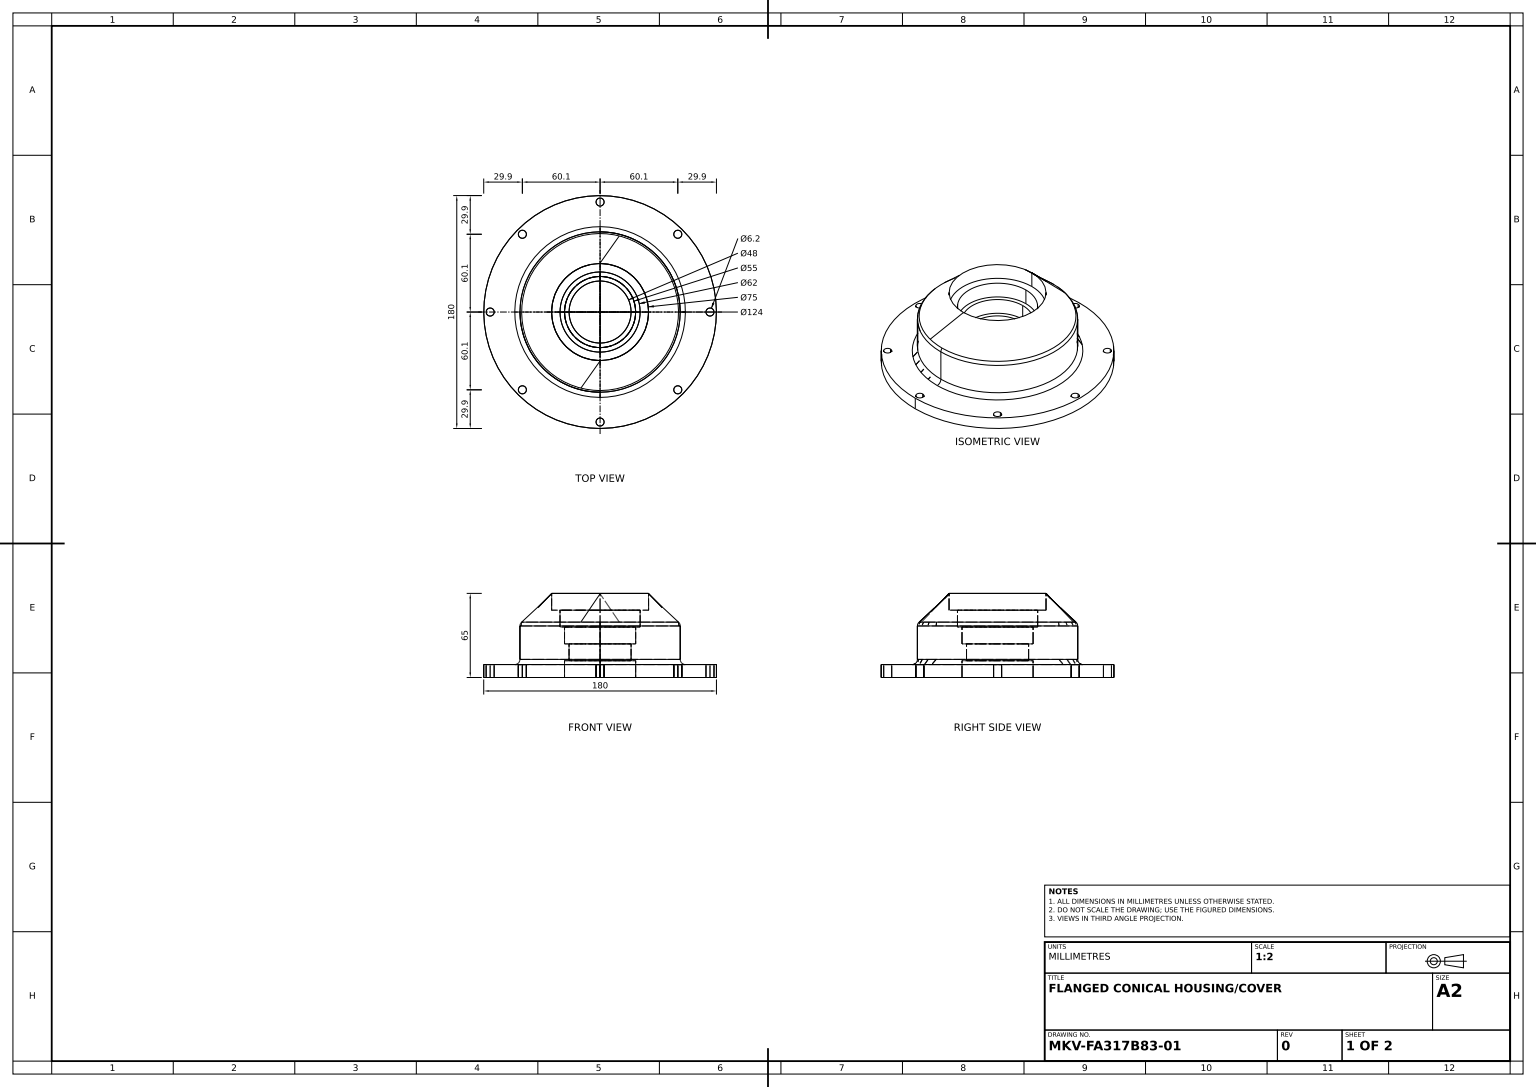
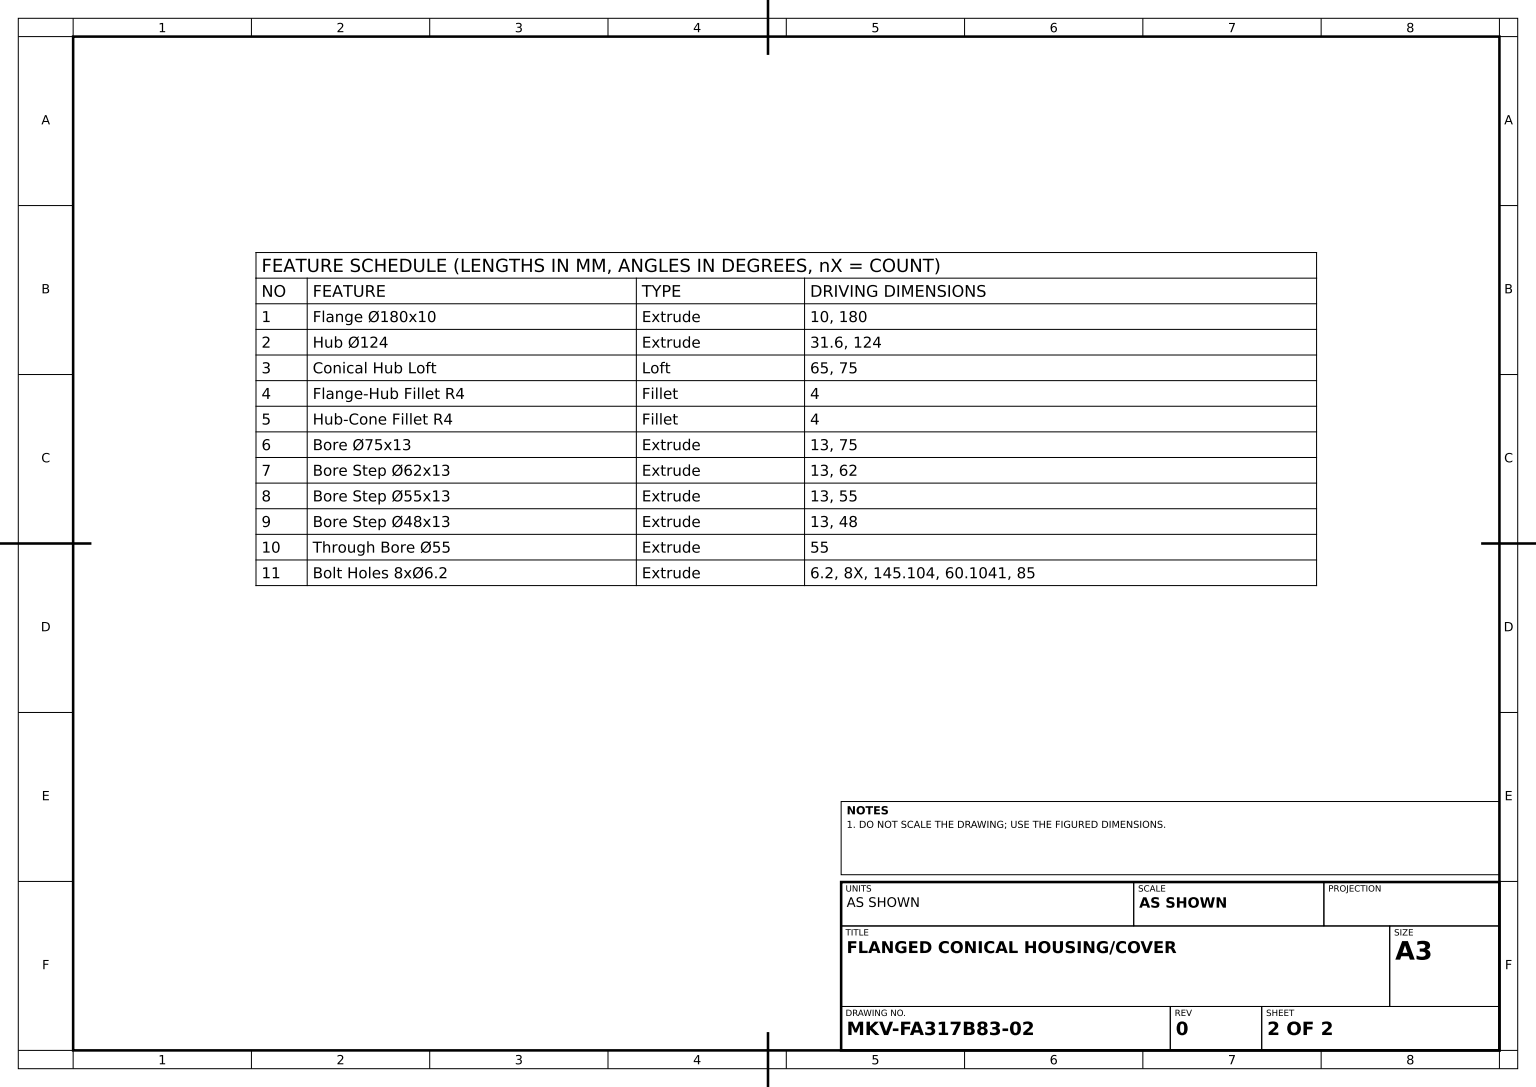
ISO-10303-21;
HEADER;
FILE_DESCRIPTION((''),'2;1');
FILE_NAME('','',(''),(''),'','','');
FILE_SCHEMA(('AUTOMOTIVE_DESIGN'));
ENDSEC;
DATA;
#1=APPLICATION_CONTEXT('');
#2=PRODUCT_CONTEXT('',#1,'mechanical');
#3=PRODUCT('','','',(#2));
#4=PRODUCT_DEFINITION_FORMATION('','',#3);
#5=PRODUCT_DEFINITION_CONTEXT('',#1,'design');
#6=PRODUCT_DEFINITION('','',#4,#5);
#7=PRODUCT_DEFINITION_SHAPE('','',#6);
#8=(LENGTH_UNIT()NAMED_UNIT(*)SI_UNIT(.MILLI.,.METRE.));
#9=(NAMED_UNIT(*)PLANE_ANGLE_UNIT()SI_UNIT($,.RADIAN.));
#10=(NAMED_UNIT(*)SI_UNIT($,.STERADIAN.)SOLID_ANGLE_UNIT());
#11=UNCERTAINTY_MEASURE_WITH_UNIT(LENGTH_MEASURE(1.E-05),#8,'distance_accuracy_value','');
#12=(GEOMETRIC_REPRESENTATION_CONTEXT(3)GLOBAL_UNCERTAINTY_ASSIGNED_CONTEXT((#11))GLOBAL_UNIT_ASSIGNED_CONTEXT((#8,#9,#10))REPRESENTATION_CONTEXT('',''));
#13=CARTESIAN_POINT('',(60.104076,10.,-63.204076));
#14=VERTEX_POINT('',#13);
#15=CARTESIAN_POINT('',(60.104076,10.,-57.004076));
#16=VERTEX_POINT('',#15);
#17=CARTESIAN_POINT('',(60.104076,10.,-60.104076));
#18=DIRECTION('',(0.,1.,0.));
#19=DIRECTION('',(0.,0.,1.));
#20=AXIS2_PLACEMENT_3D('',#17,#18,#19);
#21=CIRCLE('',#20,3.1);
#22=EDGE_CURVE('',#14,#16,#21,.T.);
#23=ORIENTED_EDGE('',*,*,#22,.T.);
#24=CARTESIAN_POINT('',(60.104076,0.,-57.004076));
#25=VERTEX_POINT('',#24);
#26=VECTOR('',#18,1000.);
#27=LINE('',#24,#26);
#28=EDGE_CURVE('',#25,#16,#27,.T.);
#29=ORIENTED_EDGE('',*,*,#28,.F.);
#30=CARTESIAN_POINT('',(60.104076,0.,-63.204076));
#31=VERTEX_POINT('',#30);
#32=CARTESIAN_POINT('',(60.104076,0.,-60.104076));
#33=AXIS2_PLACEMENT_3D('',#32,#18,#19);
#34=CIRCLE('',#33,3.1);
#35=EDGE_CURVE('',#31,#25,#34,.T.);
#36=ORIENTED_EDGE('',*,*,#35,.F.);
#37=LINE('',#30,#26);
#38=EDGE_CURVE('',#31,#14,#37,.T.);
#39=ORIENTED_EDGE('',*,*,#38,.T.);
#40=EDGE_LOOP('',(#23,#29,#36,#39));
#41=FACE_OUTER_BOUND('',#40,.T.);
#42=CYLINDRICAL_SURFACE('',#33,3.1);
#43=ADVANCED_FACE('',(#41),#42,.F.);
#44=CARTESIAN_POINT('',(60.104076,0.,57.004076));
#45=VERTEX_POINT('',#44);
#46=CARTESIAN_POINT('',(60.104076,10.,57.004076));
#47=VERTEX_POINT('',#46);
#48=LINE('',#44,#26);
#49=EDGE_CURVE('',#45,#47,#48,.T.);
#50=ORIENTED_EDGE('',*,*,#49,.T.);
#51=CARTESIAN_POINT('',(60.104076,10.,63.204076));
#52=VERTEX_POINT('',#51);
#53=CARTESIAN_POINT('',(60.104076,10.,60.104076));
#54=AXIS2_PLACEMENT_3D('',#53,#18,#19);
#55=CIRCLE('',#54,3.1);
#56=EDGE_CURVE('',#47,#52,#55,.T.);
#57=ORIENTED_EDGE('',*,*,#56,.T.);
#58=CARTESIAN_POINT('',(60.104076,0.,63.204076));
#59=VERTEX_POINT('',#58);
#60=LINE('',#58,#26);
#61=EDGE_CURVE('',#59,#52,#60,.T.);
#62=ORIENTED_EDGE('',*,*,#61,.F.);
#63=CARTESIAN_POINT('',(60.104076,0.,60.104076));
#64=AXIS2_PLACEMENT_3D('',#63,#18,#19);
#65=CIRCLE('',#64,3.1);
#66=EDGE_CURVE('',#45,#59,#65,.T.);
#67=ORIENTED_EDGE('',*,*,#66,.F.);
#68=EDGE_LOOP('',(#50,#57,#62,#67));
#69=FACE_OUTER_BOUND('',#68,.T.);
#70=CYLINDRICAL_SURFACE('',#64,3.1);
#71=ADVANCED_FACE('',(#69),#70,.F.);
#72=CARTESIAN_POINT('',(0.,14.,-62.));
#73=VERTEX_POINT('',#72);
#74=CARTESIAN_POINT('',(0.,10.,-66.));
#75=VERTEX_POINT('',#74);
#76=CARTESIAN_POINT('',(0.,14.,-66.));
#77=DIRECTION('',(1.,0.,0.));
#78=DIRECTION('',(0.,0.,-1.));
#79=AXIS2_PLACEMENT_3D('',#76,#77,#78);
#80=CIRCLE('',#79,4.);
#81=EDGE_CURVE('',#73,#75,#80,.T.);
#82=ORIENTED_EDGE('',*,*,#81,.F.);
#83=CARTESIAN_POINT('',(0.,14.,62.));
#84=VERTEX_POINT('',#83);
#85=CARTESIAN_POINT('',(0.,14.,0.));
#86=AXIS2_PLACEMENT_3D('',#85,#18,#19);
#87=CIRCLE('',#86,62.);
#88=EDGE_CURVE('',#84,#73,#87,.T.);
#89=ORIENTED_EDGE('',*,*,#88,.F.);
#90=CARTESIAN_POINT('',(0.,10.,66.));
#91=VERTEX_POINT('',#90);
#92=CARTESIAN_POINT('',(0.,14.,66.));
#93=DIRECTION('',(-1.,0.,0.));
#94=AXIS2_PLACEMENT_3D('',#92,#93,#19);
#95=CIRCLE('',#94,4.);
#96=EDGE_CURVE('',#84,#91,#95,.T.);
#97=ORIENTED_EDGE('',*,*,#96,.T.);
#98=CARTESIAN_POINT('',(0.,10.,0.));
#99=DIRECTION('',(0.,-1.,0.));
#100=AXIS2_PLACEMENT_3D('',#98,#99,#19);
#101=CIRCLE('',#100,66.);
#102=EDGE_CURVE('',#75,#91,#101,.T.);
#103=ORIENTED_EDGE('',*,*,#102,.F.);
#104=EDGE_LOOP('',(#82,#89,#97,#103));
#105=FACE_OUTER_BOUND('',#104,.T.);
#106=TOROIDAL_SURFACE('',#86,66.,4.);
#107=ADVANCED_FACE('',(#105),#106,.F.);
#108=EDGE_CURVE('',#16,#14,#21,.T.);
#109=ORIENTED_EDGE('',*,*,#108,.T.);
#110=ORIENTED_EDGE('',*,*,#38,.F.);
#111=EDGE_CURVE('',#25,#31,#34,.T.);
#112=ORIENTED_EDGE('',*,*,#111,.F.);
#113=ORIENTED_EDGE('',*,*,#28,.T.);
#114=EDGE_LOOP('',(#109,#110,#112,#113));
#115=FACE_OUTER_BOUND('',#114,.T.);
#116=ADVANCED_FACE('',(#115),#42,.F.);
#117=CARTESIAN_POINT('',(0.,10.,90.));
#118=VERTEX_POINT('',#117);
#119=CARTESIAN_POINT('',(0.,10.,-90.));
#120=VERTEX_POINT('',#119);
#121=AXIS2_PLACEMENT_3D('',#98,#18,#19);
#122=CIRCLE('',#121,90.);
#123=EDGE_CURVE('',#118,#120,#122,.T.);
#124=ORIENTED_EDGE('',*,*,#123,.F.);
#125=CARTESIAN_POINT('',(0.,0.,90.));
#126=VERTEX_POINT('',#125);
#127=VECTOR('',#99,1000.);
#128=LINE('',#117,#127);
#129=EDGE_CURVE('',#118,#126,#128,.T.);
#130=ORIENTED_EDGE('',*,*,#129,.T.);
#131=CARTESIAN_POINT('',(0.,0.,-90.));
#132=VERTEX_POINT('',#131);
#133=CARTESIAN_POINT('',(0.,0.,0.));
#134=AXIS2_PLACEMENT_3D('',#133,#18,#19);
#135=CIRCLE('',#134,90.);
#136=EDGE_CURVE('',#126,#132,#135,.T.);
#137=ORIENTED_EDGE('',*,*,#136,.T.);
#138=LINE('',#119,#127);
#139=EDGE_CURVE('',#120,#132,#138,.T.);
#140=ORIENTED_EDGE('',*,*,#139,.F.);
#141=EDGE_LOOP('',(#124,#130,#137,#140));
#142=FACE_OUTER_BOUND('',#141,.T.);
#143=AXIS2_PLACEMENT_3D('',#98,#99,#78);
#144=CYLINDRICAL_SURFACE('',#143,90.);
#145=ADVANCED_FACE('',(#142),#144,.T.);
#146=CARTESIAN_POINT('',(0.,52.,37.5));
#147=VERTEX_POINT('',#146);
#148=CARTESIAN_POINT('',(0.,65.,37.5));
#149=VERTEX_POINT('',#148);
#150=LINE('',#146,#26);
#151=EDGE_CURVE('',#147,#149,#150,.T.);
#152=ORIENTED_EDGE('',*,*,#151,.T.);
#153=CARTESIAN_POINT('',(0.212056,65.,37.4994));
#154=VERTEX_POINT('',#153);
#155=CARTESIAN_POINT('',(0.035343,65.,37.5));
#156=CARTESIAN_POINT('',(0.106029,65.,37.4999));
#157=CARTESIAN_POINT('',(0.176714,65.,37.4996));
#158=B_SPLINE_CURVE_WITH_KNOTS('',3,(#148,#155,#156,#157,#153),.UNSPECIFIED.,.F.,.F.,(4,1,4),(0.,0.00045,0.0009),.UNSPECIFIED.);
#159=EDGE_CURVE('',#149,#154,#158,.T.);
#160=ORIENTED_EDGE('',*,*,#159,.T.);
#161=CARTESIAN_POINT('',(0.,65.,-37.5));
#162=VERTEX_POINT('',#161);
#163=CARTESIAN_POINT('',(2.661969,65.,37.485546));
#164=CARTESIAN_POINT('',(5.110459,65.,37.23084));
#165=CARTESIAN_POINT('',(9.911076,65.,36.249453));
#166=CARTESIAN_POINT('',(12.263085,65.,35.522796));
#167=CARTESIAN_POINT('',(16.780672,65.,33.625308));
#168=CARTESIAN_POINT('',(18.946138,65.,32.454524));
#169=CARTESIAN_POINT('',(23.007708,65.,29.713594));
#170=CARTESIAN_POINT('',(24.903712,65.,28.143515));
#171=CARTESIAN_POINT('',(28.35374,65.,24.664097));
#172=CARTESIAN_POINT('',(29.907681,65.,22.754843));
#173=CARTESIAN_POINT('',(32.614061,65.,18.670171));
#174=CARTESIAN_POINT('',(33.766435,65.,16.494852));
#175=CARTESIAN_POINT('',(35.625536,65.,11.961333));
#176=CARTESIAN_POINT('',(36.332217,65.,9.603244));
#177=CARTESIAN_POINT('',(37.272849,65.,4.794475));
#178=CARTESIAN_POINT('',(37.506777,65.,2.343913));
#179=CARTESIAN_POINT('',(37.492923,65.,-2.55597));
#180=CARTESIAN_POINT('',(37.245141,65.,-5.005171));
#181=CARTESIAN_POINT('',(36.277331,65.,-9.808544));
#182=CARTESIAN_POINT('',(35.557327,65.,-12.162598));
#183=CARTESIAN_POINT('',(33.672619,65.,-16.685531));
#184=CARTESIAN_POINT('',(32.507963,65.,-18.854299));
#185=CARTESIAN_POINT('',(29.778528,65.,-22.923603));
#186=CARTESIAN_POINT('',(28.213816,65.,-24.824038));
#187=CARTESIAN_POINT('',(24.744166,65.,-28.283891));
#188=CARTESIAN_POINT('',(22.839314,65.,-29.843223));
#189=CARTESIAN_POINT('',(18.76231,65.,-32.561142));
#190=CARTESIAN_POINT('',(16.590258,65.,-33.719662));
#191=CARTESIAN_POINT('',(12.062014,65.,-35.591573));
#192=CARTESIAN_POINT('',(9.705933,65.,-36.304919));
#193=CARTESIAN_POINT('',(4.899843,65.,-37.259144));
#194=CARTESIAN_POINT('',(2.449951,65.,-37.5));
#195=B_SPLINE_CURVE_WITH_KNOTS('',3,(#153,#163,#164,#165,#166,#167,#168,#169,#170,#171,#172,#173,#174,#175,#176,#177,#178,#179,#180,#181,#182,#183,#184,#185,#186,#187,#188,#189,#190,#191,#192,#193,#194,#161),.UNSPECIFIED.,.F.,.F.,(4,2,2,2,2,2,2,2,2,2,2,2,2,2,2,2,4),(0.0009,0.03209375,0.0632875,0.09448125,0.125675,0.15686875,0.1880625,0.21925625,0.25045,0.28164375,0.3128375,0.34403125,0.375225,0.40641875,0.4376125,0.46880625,0.5),.UNSPECIFIED.);
#196=EDGE_CURVE('',#154,#162,#195,.T.);
#197=ORIENTED_EDGE('',*,*,#196,.T.);
#198=CARTESIAN_POINT('',(0.,52.,-37.5));
#199=VERTEX_POINT('',#198);
#200=LINE('',#198,#26);
#201=EDGE_CURVE('',#199,#162,#200,.T.);
#202=ORIENTED_EDGE('',*,*,#201,.F.);
#203=CARTESIAN_POINT('',(0.,52.,0.));
#204=AXIS2_PLACEMENT_3D('',#203,#18,#19);
#205=CIRCLE('',#204,37.5);
#206=EDGE_CURVE('',#147,#199,#205,.T.);
#207=ORIENTED_EDGE('',*,*,#206,.F.);
#208=EDGE_LOOP('',(#152,#160,#197,#202,#207));
#209=FACE_OUTER_BOUND('',#208,.T.);
#210=CYLINDRICAL_SURFACE('',#204,37.5);
#211=ADVANCED_FACE('',(#209),#210,.F.);
#212=CARTESIAN_POINT('',(85.,0.,-3.1));
#213=VERTEX_POINT('',#212);
#214=CARTESIAN_POINT('',(85.,0.,3.1));
#215=VERTEX_POINT('',#214);
#216=CARTESIAN_POINT('',(85.,0.,0.));
#217=AXIS2_PLACEMENT_3D('',#216,#18,#19);
#218=CIRCLE('',#217,3.1);
#219=EDGE_CURVE('',#213,#215,#218,.T.);
#220=ORIENTED_EDGE('',*,*,#219,.F.);
#221=CARTESIAN_POINT('',(85.,10.,-3.1));
#222=VERTEX_POINT('',#221);
#223=LINE('',#212,#26);
#224=EDGE_CURVE('',#213,#222,#223,.T.);
#225=ORIENTED_EDGE('',*,*,#224,.T.);
#226=CARTESIAN_POINT('',(85.,10.,3.1));
#227=VERTEX_POINT('',#226);
#228=CARTESIAN_POINT('',(85.,10.,0.));
#229=AXIS2_PLACEMENT_3D('',#228,#18,#19);
#230=CIRCLE('',#229,3.1);
#231=EDGE_CURVE('',#222,#227,#230,.T.);
#232=ORIENTED_EDGE('',*,*,#231,.T.);
#233=LINE('',#214,#26);
#234=EDGE_CURVE('',#215,#227,#233,.T.);
#235=ORIENTED_EDGE('',*,*,#234,.F.);
#236=EDGE_LOOP('',(#220,#225,#232,#235));
#237=FACE_OUTER_BOUND('',#236,.T.);
#238=CYLINDRICAL_SURFACE('',#217,3.1);
#239=ADVANCED_FACE('',(#237),#238,.F.);
#240=CARTESIAN_POINT('',(0.,26.,27.5));
#241=VERTEX_POINT('',#240);
#242=CARTESIAN_POINT('',(0.,39.,27.5));
#243=VERTEX_POINT('',#242);
#244=LINE('',#240,#26);
#245=EDGE_CURVE('',#241,#243,#244,.T.);
#246=ORIENTED_EDGE('',*,*,#245,.T.);
#247=CARTESIAN_POINT('',(0.,39.,-27.5));
#248=VERTEX_POINT('',#247);
#249=CARTESIAN_POINT('',(0.,39.,0.));
#250=AXIS2_PLACEMENT_3D('',#249,#18,#19);
#251=CIRCLE('',#250,27.5);
#252=EDGE_CURVE('',#243,#248,#251,.T.);
#253=ORIENTED_EDGE('',*,*,#252,.T.);
#254=CARTESIAN_POINT('',(0.,26.,-27.5));
#255=VERTEX_POINT('',#254);
#256=LINE('',#254,#26);
#257=EDGE_CURVE('',#255,#248,#256,.T.);
#258=ORIENTED_EDGE('',*,*,#257,.F.);
#259=CARTESIAN_POINT('',(0.,26.,0.));
#260=AXIS2_PLACEMENT_3D('',#259,#18,#19);
#261=CIRCLE('',#260,27.5);
#262=EDGE_CURVE('',#241,#255,#261,.T.);
#263=ORIENTED_EDGE('',*,*,#262,.F.);
#264=EDGE_LOOP('',(#246,#253,#258,#263));
#265=FACE_OUTER_BOUND('',#264,.T.);
#266=CYLINDRICAL_SURFACE('',#260,27.5);
#267=ADVANCED_FACE('',(#265),#266,.F.);
#268=CARTESIAN_POINT('',(0.,39.,31.));
#269=VERTEX_POINT('',#268);
#270=CARTESIAN_POINT('',(0.,39.,-31.));
#271=VERTEX_POINT('',#270);
#272=CIRCLE('',#250,31.);
#273=EDGE_CURVE('',#269,#271,#272,.T.);
#274=ORIENTED_EDGE('',*,*,#273,.T.);
#275=EDGE_CURVE('',#271,#269,#272,.T.);
#276=ORIENTED_EDGE('',*,*,#275,.T.);
#277=EDGE_LOOP('',(#274,#276));
#278=FACE_OUTER_BOUND('',#277,.T.);
#279=ORIENTED_EDGE('',*,*,#252,.F.);
#280=EDGE_CURVE('',#248,#243,#251,.T.);
#281=ORIENTED_EDGE('',*,*,#280,.F.);
#282=EDGE_LOOP('',(#279,#281));
#283=FACE_BOUND('',#282,.T.);
#284=PLANE('',#250);
#285=ADVANCED_FACE('',(#278,#283),#284,.T.);
#286=CARTESIAN_POINT('',(-60.104076,0.,63.204076));
#287=VERTEX_POINT('',#286);
#288=CARTESIAN_POINT('',(-60.104076,10.,63.204076));
#289=VERTEX_POINT('',#288);
#290=LINE('',#286,#26);
#291=EDGE_CURVE('',#287,#289,#290,.T.);
#292=ORIENTED_EDGE('',*,*,#291,.T.);
#293=CARTESIAN_POINT('',(-60.104076,10.,57.004076));
#294=VERTEX_POINT('',#293);
#295=CARTESIAN_POINT('',(-60.104076,10.,60.104076));
#296=AXIS2_PLACEMENT_3D('',#295,#18,#19);
#297=CIRCLE('',#296,3.1);
#298=EDGE_CURVE('',#289,#294,#297,.T.);
#299=ORIENTED_EDGE('',*,*,#298,.T.);
#300=CARTESIAN_POINT('',(-60.104076,0.,57.004076));
#301=VERTEX_POINT('',#300);
#302=LINE('',#300,#26);
#303=EDGE_CURVE('',#301,#294,#302,.T.);
#304=ORIENTED_EDGE('',*,*,#303,.F.);
#305=CARTESIAN_POINT('',(-60.104076,0.,60.104076));
#306=AXIS2_PLACEMENT_3D('',#305,#18,#19);
#307=CIRCLE('',#306,3.1);
#308=EDGE_CURVE('',#287,#301,#307,.T.);
#309=ORIENTED_EDGE('',*,*,#308,.F.);
#310=EDGE_LOOP('',(#292,#299,#304,#309));
#311=FACE_OUTER_BOUND('',#310,.T.);
#312=CYLINDRICAL_SURFACE('',#306,3.1);
#313=ADVANCED_FACE('',(#311),#312,.F.);
#314=CARTESIAN_POINT('',(0.,0.,88.1));
#315=VERTEX_POINT('',#314);
#316=CARTESIAN_POINT('',(0.,10.,88.1));
#317=VERTEX_POINT('',#316);
#318=LINE('',#314,#26);
#319=EDGE_CURVE('',#315,#317,#318,.T.);
#320=ORIENTED_EDGE('',*,*,#319,.F.);
#321=CARTESIAN_POINT('',(0.,0.,81.9));
#322=VERTEX_POINT('',#321);
#323=CARTESIAN_POINT('',(0.,0.,85.));
#324=AXIS2_PLACEMENT_3D('',#323,#18,#19);
#325=CIRCLE('',#324,3.1);
#326=EDGE_CURVE('',#322,#315,#325,.T.);
#327=ORIENTED_EDGE('',*,*,#326,.F.);
#328=CARTESIAN_POINT('',(0.,10.,81.9));
#329=VERTEX_POINT('',#328);
#330=LINE('',#321,#26);
#331=EDGE_CURVE('',#322,#329,#330,.T.);
#332=ORIENTED_EDGE('',*,*,#331,.T.);
#333=CARTESIAN_POINT('',(0.,10.,85.));
#334=AXIS2_PLACEMENT_3D('',#333,#18,#19);
#335=CIRCLE('',#334,3.1);
#336=EDGE_CURVE('',#329,#317,#335,.T.);
#337=ORIENTED_EDGE('',*,*,#336,.T.);
#338=EDGE_LOOP('',(#320,#327,#332,#337));
#339=FACE_OUTER_BOUND('',#338,.T.);
#340=CYLINDRICAL_SURFACE('',#324,3.1);
#341=ADVANCED_FACE('',(#339),#340,.F.);
#342=ORIENTED_EDGE('',*,*,#303,.T.);
#343=EDGE_CURVE('',#294,#289,#297,.T.);
#344=ORIENTED_EDGE('',*,*,#343,.T.);
#345=ORIENTED_EDGE('',*,*,#291,.F.);
#346=EDGE_CURVE('',#301,#287,#307,.T.);
#347=ORIENTED_EDGE('',*,*,#346,.F.);
#348=EDGE_LOOP('',(#342,#344,#345,#347));
#349=FACE_OUTER_BOUND('',#348,.T.);
#350=ADVANCED_FACE('',(#349),#312,.F.);
#351=CARTESIAN_POINT('',(0.,13.,-24.));
#352=VERTEX_POINT('',#351);
#353=CARTESIAN_POINT('',(0.,26.,-24.));
#354=VERTEX_POINT('',#353);
#355=LINE('',#351,#26);
#356=EDGE_CURVE('',#352,#354,#355,.T.);
#357=ORIENTED_EDGE('',*,*,#356,.F.);
#358=CARTESIAN_POINT('',(0.,13.,24.));
#359=VERTEX_POINT('',#358);
#360=CARTESIAN_POINT('',(0.,13.,0.));
#361=AXIS2_PLACEMENT_3D('',#360,#18,#19);
#362=CIRCLE('',#361,24.);
#363=EDGE_CURVE('',#359,#352,#362,.T.);
#364=ORIENTED_EDGE('',*,*,#363,.F.);
#365=CARTESIAN_POINT('',(0.,26.,24.));
#366=VERTEX_POINT('',#365);
#367=LINE('',#358,#26);
#368=EDGE_CURVE('',#359,#366,#367,.T.);
#369=ORIENTED_EDGE('',*,*,#368,.T.);
#370=CIRCLE('',#260,24.);
#371=EDGE_CURVE('',#366,#354,#370,.T.);
#372=ORIENTED_EDGE('',*,*,#371,.T.);
#373=EDGE_LOOP('',(#357,#364,#369,#372));
#374=FACE_OUTER_BOUND('',#373,.T.);
#375=CYLINDRICAL_SURFACE('',#361,24.);
#376=ADVANCED_FACE('',(#374),#375,.F.);
#377=CARTESIAN_POINT('',(0.,0.,27.5));
#378=VERTEX_POINT('',#377);
#379=CARTESIAN_POINT('',(0.,13.,27.5));
#380=VERTEX_POINT('',#379);
#381=LINE('',#377,#26);
#382=EDGE_CURVE('',#378,#380,#381,.T.);
#383=ORIENTED_EDGE('',*,*,#382,.F.);
#384=CARTESIAN_POINT('',(0.,0.,-27.5));
#385=VERTEX_POINT('',#384);
#386=CIRCLE('',#134,27.5);
#387=EDGE_CURVE('',#385,#378,#386,.T.);
#388=ORIENTED_EDGE('',*,*,#387,.F.);
#389=CARTESIAN_POINT('',(0.,13.,-27.5));
#390=VERTEX_POINT('',#389);
#391=LINE('',#384,#26);
#392=EDGE_CURVE('',#385,#390,#391,.T.);
#393=ORIENTED_EDGE('',*,*,#392,.T.);
#394=CIRCLE('',#361,27.5);
#395=EDGE_CURVE('',#390,#380,#394,.T.);
#396=ORIENTED_EDGE('',*,*,#395,.T.);
#397=EDGE_LOOP('',(#383,#388,#393,#396));
#398=FACE_OUTER_BOUND('',#397,.T.);
#399=CYLINDRICAL_SURFACE('',#134,27.5);
#400=ADVANCED_FACE('',(#398),#399,.F.);
#401=CARTESIAN_POINT('',(0.,52.,31.));
#402=VERTEX_POINT('',#401);
#403=CARTESIAN_POINT('',(0.,52.,-31.));
#404=VERTEX_POINT('',#403);
#405=CIRCLE('',#204,31.);
#406=EDGE_CURVE('',#402,#404,#405,.T.);
#407=ORIENTED_EDGE('',*,*,#406,.F.);
#408=EDGE_CURVE('',#404,#402,#405,.T.);
#409=ORIENTED_EDGE('',*,*,#408,.F.);
#410=EDGE_LOOP('',(#407,#409));
#411=FACE_BOUND('',#410,.T.);
#412=ORIENTED_EDGE('',*,*,#206,.T.);
#413=EDGE_CURVE('',#199,#147,#205,.T.);
#414=ORIENTED_EDGE('',*,*,#413,.T.);
#415=EDGE_LOOP('',(#412,#414));
#416=FACE_OUTER_BOUND('',#415,.T.);
#417=PLANE('',#204);
#418=ADVANCED_FACE('',(#411,#416),#417,.T.);
#419=EDGE_CURVE('',#59,#45,#65,.T.);
#420=ORIENTED_EDGE('',*,*,#419,.T.);
#421=ORIENTED_EDGE('',*,*,#66,.T.);
#422=EDGE_LOOP('',(#420,#421));
#423=FACE_BOUND('',#422,.T.);
#424=CARTESIAN_POINT('',(-60.104076,0.,-63.204076));
#425=VERTEX_POINT('',#424);
#426=CARTESIAN_POINT('',(-60.104076,0.,-57.004076));
#427=VERTEX_POINT('',#426);
#428=CARTESIAN_POINT('',(-60.104076,0.,-60.104076));
#429=AXIS2_PLACEMENT_3D('',#428,#18,#19);
#430=CIRCLE('',#429,3.1);
#431=EDGE_CURVE('',#425,#427,#430,.T.);
#432=ORIENTED_EDGE('',*,*,#431,.T.);
#433=EDGE_CURVE('',#427,#425,#430,.T.);
#434=ORIENTED_EDGE('',*,*,#433,.T.);
#435=EDGE_LOOP('',(#432,#434));
#436=FACE_BOUND('',#435,.T.);
#437=CARTESIAN_POINT('',(0.,0.,-88.1));
#438=VERTEX_POINT('',#437);
#439=CARTESIAN_POINT('',(0.,0.,-81.9));
#440=VERTEX_POINT('',#439);
#441=CARTESIAN_POINT('',(0.,0.,-85.));
#442=AXIS2_PLACEMENT_3D('',#441,#18,#19);
#443=CIRCLE('',#442,3.1);
#444=EDGE_CURVE('',#438,#440,#443,.T.);
#445=ORIENTED_EDGE('',*,*,#444,.T.);
#446=EDGE_CURVE('',#440,#438,#443,.T.);
#447=ORIENTED_EDGE('',*,*,#446,.T.);
#448=EDGE_LOOP('',(#445,#447));
#449=FACE_BOUND('',#448,.T.);
#450=ORIENTED_EDGE('',*,*,#387,.T.);
#451=EDGE_CURVE('',#378,#385,#386,.T.);
#452=ORIENTED_EDGE('',*,*,#451,.T.);
#453=EDGE_LOOP('',(#450,#452));
#454=FACE_BOUND('',#453,.T.);
#455=EDGE_CURVE('',#315,#322,#325,.T.);
#456=ORIENTED_EDGE('',*,*,#455,.T.);
#457=ORIENTED_EDGE('',*,*,#326,.T.);
#458=EDGE_LOOP('',(#456,#457));
#459=FACE_BOUND('',#458,.T.);
#460=ORIENTED_EDGE('',*,*,#35,.T.);
#461=ORIENTED_EDGE('',*,*,#111,.T.);
#462=EDGE_LOOP('',(#460,#461));
#463=FACE_BOUND('',#462,.T.);
#464=ORIENTED_EDGE('',*,*,#308,.T.);
#465=ORIENTED_EDGE('',*,*,#346,.T.);
#466=EDGE_LOOP('',(#464,#465));
#467=FACE_BOUND('',#466,.T.);
#468=CARTESIAN_POINT('',(-85.,0.,3.1));
#469=VERTEX_POINT('',#468);
#470=CARTESIAN_POINT('',(-85.,0.,-3.1));
#471=VERTEX_POINT('',#470);
#472=CARTESIAN_POINT('',(-85.,0.,0.));
#473=AXIS2_PLACEMENT_3D('',#472,#18,#19);
#474=CIRCLE('',#473,3.1);
#475=EDGE_CURVE('',#469,#471,#474,.T.);
#476=ORIENTED_EDGE('',*,*,#475,.T.);
#477=EDGE_CURVE('',#471,#469,#474,.T.);
#478=ORIENTED_EDGE('',*,*,#477,.T.);
#479=EDGE_LOOP('',(#476,#478));
#480=FACE_BOUND('',#479,.T.);
#481=EDGE_CURVE('',#215,#213,#218,.T.);
#482=ORIENTED_EDGE('',*,*,#481,.T.);
#483=ORIENTED_EDGE('',*,*,#219,.T.);
#484=EDGE_LOOP('',(#482,#483));
#485=FACE_BOUND('',#484,.T.);
#486=EDGE_CURVE('',#132,#126,#135,.T.);
#487=ORIENTED_EDGE('',*,*,#486,.F.);
#488=ORIENTED_EDGE('',*,*,#136,.F.);
#489=EDGE_LOOP('',(#487,#488));
#490=FACE_OUTER_BOUND('',#489,.T.);
#491=PLANE('',#134);
#492=ADVANCED_FACE('',(#423,#436,#449,#454,#459,#463,#467,#480,#485,#490),#491,.F.);
#493=ORIENTED_EDGE('',*,*,#371,.F.);
#494=EDGE_CURVE('',#354,#366,#370,.T.);
#495=ORIENTED_EDGE('',*,*,#494,.F.);
#496=EDGE_LOOP('',(#493,#495));
#497=FACE_BOUND('',#496,.T.);
#498=EDGE_CURVE('',#255,#241,#261,.T.);
#499=ORIENTED_EDGE('',*,*,#498,.T.);
#500=ORIENTED_EDGE('',*,*,#262,.T.);
#501=EDGE_LOOP('',(#499,#500));
#502=FACE_OUTER_BOUND('',#501,.T.);
#503=PLANE('',#260);
#504=ADVANCED_FACE('',(#497,#502),#503,.T.);
#505=CARTESIAN_POINT('',(-85.,10.,3.1));
#506=VERTEX_POINT('',#505);
#507=CARTESIAN_POINT('',(-85.,10.,-3.1));
#508=VERTEX_POINT('',#507);
#509=CARTESIAN_POINT('',(-85.,10.,0.));
#510=AXIS2_PLACEMENT_3D('',#509,#18,#19);
#511=CIRCLE('',#510,3.1);
#512=EDGE_CURVE('',#506,#508,#511,.T.);
#513=ORIENTED_EDGE('',*,*,#512,.T.);
#514=LINE('',#470,#26);
#515=EDGE_CURVE('',#471,#508,#514,.T.);
#516=ORIENTED_EDGE('',*,*,#515,.F.);
#517=ORIENTED_EDGE('',*,*,#475,.F.);
#518=LINE('',#468,#26);
#519=EDGE_CURVE('',#469,#506,#518,.T.);
#520=ORIENTED_EDGE('',*,*,#519,.T.);
#521=EDGE_LOOP('',(#513,#516,#517,#520));
#522=FACE_OUTER_BOUND('',#521,.T.);
#523=CYLINDRICAL_SURFACE('',#473,3.1);
#524=ADVANCED_FACE('',(#522),#523,.F.);
#525=CARTESIAN_POINT('',(0.,42.788159,60.693308));
#526=VERTEX_POINT('',#525);
#527=CARTESIAN_POINT('',(14.875671,42.788159,-58.842094));
#528=VERTEX_POINT('',#527);
#529=CARTESIAN_POINT('',(0.,42.788159,0.));
#530=AXIS2_PLACEMENT_3D('',#529,#18,#19);
#531=CIRCLE('',#530,60.693308);
#532=EDGE_CURVE('',#526,#528,#531,.T.);
#533=ORIENTED_EDGE('',*,*,#532,.F.);
#534=CARTESIAN_POINT('',(0.,39.830779,62.));
#535=VERTEX_POINT('',#534);
#536=CARTESIAN_POINT('',(0.,39.830779,58.));
#537=AXIS2_PLACEMENT_3D('',#536,#77,#78);
#538=CIRCLE('',#537,4.);
#539=EDGE_CURVE('',#526,#535,#538,.T.);
#540=ORIENTED_EDGE('',*,*,#539,.T.);
#541=CARTESIAN_POINT('',(0.,39.830779,-62.));
#542=VERTEX_POINT('',#541);
#543=CARTESIAN_POINT('',(0.,39.830779,0.));
#544=AXIS2_PLACEMENT_3D('',#543,#99,#78);
#545=CIRCLE('',#544,62.);
#546=EDGE_CURVE('',#542,#535,#545,.T.);
#547=ORIENTED_EDGE('',*,*,#546,.F.);
#548=CARTESIAN_POINT('',(0.,42.788159,-60.693308));
#549=VERTEX_POINT('',#548);
#550=CARTESIAN_POINT('',(0.,39.830779,-58.));
#551=AXIS2_PLACEMENT_3D('',#550,#93,#19);
#552=CIRCLE('',#551,4.);
#553=EDGE_CURVE('',#549,#542,#552,.T.);
#554=ORIENTED_EDGE('',*,*,#553,.F.);
#555=EDGE_CURVE('',#528,#549,#531,.T.);
#556=ORIENTED_EDGE('',*,*,#555,.F.);
#557=EDGE_LOOP('',(#533,#540,#547,#554,#556));
#558=FACE_OUTER_BOUND('',#557,.T.);
#559=TOROIDAL_SURFACE('',#544,58.,4.);
#560=ADVANCED_FACE('',(#558),#559,.T.);
#561=ORIENTED_EDGE('',*,*,#546,.T.);
#562=CARTESIAN_POINT('',(0.,41.6,62.));
#563=LINE('',#562,#127);
#564=EDGE_CURVE('',#535,#84,#563,.T.);
#565=ORIENTED_EDGE('',*,*,#564,.T.);
#566=ORIENTED_EDGE('',*,*,#88,.T.);
#567=CARTESIAN_POINT('',(0.,41.6,-62.));
#568=LINE('',#567,#127);
#569=EDGE_CURVE('',#542,#73,#568,.T.);
#570=ORIENTED_EDGE('',*,*,#569,.F.);
#571=EDGE_LOOP('',(#561,#565,#566,#570));
#572=FACE_OUTER_BOUND('',#571,.T.);
#573=CARTESIAN_POINT('',(0.,41.6,0.));
#574=AXIS2_PLACEMENT_3D('',#573,#99,#78);
#575=CYLINDRICAL_SURFACE('',#574,62.);
#576=ADVANCED_FACE('',(#572),#575,.T.);
#577=EDGE_CURVE('',#91,#75,#101,.T.);
#578=ORIENTED_EDGE('',*,*,#577,.F.);
#579=ORIENTED_EDGE('',*,*,#96,.F.);
#580=EDGE_CURVE('',#73,#84,#87,.T.);
#581=ORIENTED_EDGE('',*,*,#580,.F.);
#582=ORIENTED_EDGE('',*,*,#81,.T.);
#583=EDGE_LOOP('',(#578,#579,#581,#582));
#584=FACE_OUTER_BOUND('',#583,.T.);
#585=ADVANCED_FACE('',(#584),#106,.F.);
#586=ORIENTED_EDGE('',*,*,#494,.T.);
#587=ORIENTED_EDGE('',*,*,#368,.F.);
#588=EDGE_CURVE('',#352,#359,#362,.T.);
#589=ORIENTED_EDGE('',*,*,#588,.F.);
#590=ORIENTED_EDGE('',*,*,#356,.T.);
#591=EDGE_LOOP('',(#586,#587,#589,#590));
#592=FACE_OUTER_BOUND('',#591,.T.);
#593=ADVANCED_FACE('',(#592),#375,.F.);
#594=CARTESIAN_POINT('',(-14.875671,42.788159,58.842094));
#595=VERTEX_POINT('',#594);
#596=EDGE_CURVE('',#549,#595,#531,.T.);
#597=ORIENTED_EDGE('',*,*,#596,.F.);
#598=ORIENTED_EDGE('',*,*,#553,.T.);
#599=EDGE_CURVE('',#535,#542,#545,.T.);
#600=ORIENTED_EDGE('',*,*,#599,.F.);
#601=ORIENTED_EDGE('',*,*,#539,.F.);
#602=EDGE_CURVE('',#595,#526,#531,.T.);
#603=ORIENTED_EDGE('',*,*,#602,.F.);
#604=EDGE_LOOP('',(#597,#598,#600,#601,#603));
#605=FACE_OUTER_BOUND('',#604,.T.);
#606=ADVANCED_FACE('',(#605),#559,.T.);
#607=ORIENTED_EDGE('',*,*,#257,.T.);
#608=ORIENTED_EDGE('',*,*,#280,.T.);
#609=ORIENTED_EDGE('',*,*,#245,.F.);
#610=ORIENTED_EDGE('',*,*,#498,.F.);
#611=EDGE_LOOP('',(#607,#608,#609,#610));
#612=FACE_OUTER_BOUND('',#611,.T.);
#613=ADVANCED_FACE('',(#612),#266,.F.);
#614=EDGE_CURVE('',#380,#390,#394,.T.);
#615=ORIENTED_EDGE('',*,*,#614,.F.);
#616=ORIENTED_EDGE('',*,*,#395,.F.);
#617=EDGE_LOOP('',(#615,#616));
#618=FACE_OUTER_BOUND('',#617,.T.);
#619=ORIENTED_EDGE('',*,*,#588,.T.);
#620=ORIENTED_EDGE('',*,*,#363,.T.);
#621=EDGE_LOOP('',(#619,#620));
#622=FACE_BOUND('',#621,.T.);
#623=PLANE('',#361);
#624=ADVANCED_FACE('',(#618,#622),#623,.F.);
#625=EDGE_CURVE('',#508,#506,#511,.T.);
#626=ORIENTED_EDGE('',*,*,#625,.T.);
#627=ORIENTED_EDGE('',*,*,#519,.F.);
#628=ORIENTED_EDGE('',*,*,#477,.F.);
#629=ORIENTED_EDGE('',*,*,#515,.T.);
#630=EDGE_LOOP('',(#626,#627,#628,#629));
#631=FACE_OUTER_BOUND('',#630,.T.);
#632=ADVANCED_FACE('',(#631),#523,.F.);
#633=ORIENTED_EDGE('',*,*,#580,.T.);
#634=ORIENTED_EDGE('',*,*,#564,.F.);
#635=ORIENTED_EDGE('',*,*,#599,.T.);
#636=ORIENTED_EDGE('',*,*,#569,.T.);
#637=EDGE_LOOP('',(#633,#634,#635,#636));
#638=FACE_OUTER_BOUND('',#637,.T.);
#639=ADVANCED_FACE('',(#638),#575,.T.);
#640=CARTESIAN_POINT('',(-60.104076,10.,-63.204076));
#641=VERTEX_POINT('',#640);
#642=LINE('',#424,#26);
#643=EDGE_CURVE('',#425,#641,#642,.T.);
#644=ORIENTED_EDGE('',*,*,#643,.T.);
#645=CARTESIAN_POINT('',(-60.104076,10.,-57.004076));
#646=VERTEX_POINT('',#645);
#647=CARTESIAN_POINT('',(-60.104076,10.,-60.104076));
#648=AXIS2_PLACEMENT_3D('',#647,#18,#19);
#649=CIRCLE('',#648,3.1);
#650=EDGE_CURVE('',#641,#646,#649,.T.);
#651=ORIENTED_EDGE('',*,*,#650,.T.);
#652=LINE('',#426,#26);
#653=EDGE_CURVE('',#427,#646,#652,.T.);
#654=ORIENTED_EDGE('',*,*,#653,.F.);
#655=ORIENTED_EDGE('',*,*,#431,.F.);
#656=EDGE_LOOP('',(#644,#651,#654,#655));
#657=FACE_OUTER_BOUND('',#656,.T.);
#658=CYLINDRICAL_SURFACE('',#429,3.1);
#659=ADVANCED_FACE('',(#657),#658,.F.);
#660=CARTESIAN_POINT('',(0.,10.,-81.9));
#661=VERTEX_POINT('',#660);
#662=LINE('',#439,#26);
#663=EDGE_CURVE('',#440,#661,#662,.T.);
#664=ORIENTED_EDGE('',*,*,#663,.F.);
#665=ORIENTED_EDGE('',*,*,#444,.F.);
#666=CARTESIAN_POINT('',(0.,10.,-88.1));
#667=VERTEX_POINT('',#666);
#668=LINE('',#437,#26);
#669=EDGE_CURVE('',#438,#667,#668,.T.);
#670=ORIENTED_EDGE('',*,*,#669,.T.);
#671=CARTESIAN_POINT('',(0.,10.,-85.));
#672=AXIS2_PLACEMENT_3D('',#671,#18,#19);
#673=CIRCLE('',#672,3.1);
#674=EDGE_CURVE('',#667,#661,#673,.T.);
#675=ORIENTED_EDGE('',*,*,#674,.T.);
#676=EDGE_LOOP('',(#664,#665,#670,#675));
#677=FACE_OUTER_BOUND('',#676,.T.);
#678=CYLINDRICAL_SURFACE('',#442,3.1);
#679=ADVANCED_FACE('',(#677),#678,.F.);
#680=B_SPLINE_CURVE_WITH_KNOTS('',1,(#594,#153),.UNSPECIFIED.,.F.,.F.,(2,2),(0.050776021,1.),.UNSPECIFIED.);
#681=EDGE_CURVE('',#595,#154,#680,.T.);
#682=ORIENTED_EDGE('',*,*,#681,.F.);
#683=ORIENTED_EDGE('',*,*,#602,.T.);
#684=ORIENTED_EDGE('',*,*,#532,.T.);
#685=CARTESIAN_POINT('',(-0.212056,65.,-37.4994));
#686=VERTEX_POINT('',#685);
#687=B_SPLINE_CURVE_WITH_KNOTS('',1,(#527,#685),.UNSPECIFIED.,.F.,.F.,(2,2),(0.050776021,1.),.UNSPECIFIED.);
#688=EDGE_CURVE('',#528,#686,#687,.T.);
#689=ORIENTED_EDGE('',*,*,#688,.T.);
#690=CARTESIAN_POINT('',(-0.035343,65.,-37.5));
#691=CARTESIAN_POINT('',(-0.106029,65.,-37.4999));
#692=CARTESIAN_POINT('',(-0.176714,65.,-37.4996));
#693=B_SPLINE_CURVE_WITH_KNOTS('',3,(#161,#690,#691,#692,#685),.UNSPECIFIED.,.F.,.F.,(4,1,4),(0.5,0.50045,0.5009),.UNSPECIFIED.);
#694=EDGE_CURVE('',#162,#686,#693,.T.);
#695=ORIENTED_EDGE('',*,*,#694,.F.);
#696=ORIENTED_EDGE('',*,*,#196,.F.);
#697=EDGE_LOOP('',(#682,#683,#684,#689,#695,#696));
#698=FACE_OUTER_BOUND('',#697,.T.);
#699=CARTESIAN_POINT('',(-15.682746,41.6,59.98376));
#700=CARTESIAN_POINT('',(104.284774,41.6,91.349252));
#701=CARTESIAN_POINT('',(75.210857,65.,37.075288));
#702=CARTESIAN_POINT('',(135.650266,41.6,-28.618268));
#703=CARTESIAN_POINT('',(74.786744,65.,-37.923513));
#704=CARTESIAN_POINT('',(15.682746,41.6,-59.98376));
#705=CARTESIAN_POINT('',(-104.284774,41.6,-91.349252));
#706=CARTESIAN_POINT('',(-75.210857,65.,-37.075288));
#707=CARTESIAN_POINT('',(-135.650266,41.6,28.618268));
#708=CARTESIAN_POINT('',(-74.786744,65.,37.923513));
#709=(BOUNDED_SURFACE()B_SPLINE_SURFACE(3,1,((#699,#153),(#700,#701),(#702,#703),(#704,#685),(#705,#706),(#707,#708),(#699,#153)),.UNSPECIFIED.,.T.,.F.,.T.)B_SPLINE_SURFACE_WITH_KNOTS((4,3,4),(2,2),(0.,0.5,1.),(0.,1.),.UNSPECIFIED.)GEOMETRIC_REPRESENTATION_ITEM()RATIONAL_B_SPLINE_SURFACE(((1.,1.),(0.333333333,0.333333333),(0.333333333,0.333333333),(1.,1.),(0.333333333,0.333333333),(0.333333333,0.333333333),(1.,1.)))REPRESENTATION_ITEM('')SURFACE());
#710=ADVANCED_FACE('',(#698),#709,.T.);
#711=LINE('',#270,#26);
#712=EDGE_CURVE('',#271,#404,#711,.T.);
#713=ORIENTED_EDGE('',*,*,#712,.F.);
#714=ORIENTED_EDGE('',*,*,#273,.F.);
#715=LINE('',#268,#26);
#716=EDGE_CURVE('',#269,#402,#715,.T.);
#717=ORIENTED_EDGE('',*,*,#716,.T.);
#718=ORIENTED_EDGE('',*,*,#406,.T.);
#719=EDGE_LOOP('',(#713,#714,#717,#718));
#720=FACE_OUTER_BOUND('',#719,.T.);
#721=CYLINDRICAL_SURFACE('',#250,31.);
#722=ADVANCED_FACE('',(#720),#721,.F.);
#723=ORIENTED_EDGE('',*,*,#22,.F.);
#724=ORIENTED_EDGE('',*,*,#108,.F.);
#725=EDGE_LOOP('',(#723,#724));
#726=FACE_BOUND('',#725,.T.);
#727=ORIENTED_EDGE('',*,*,#56,.F.);
#728=EDGE_CURVE('',#52,#47,#55,.T.);
#729=ORIENTED_EDGE('',*,*,#728,.F.);
#730=EDGE_LOOP('',(#727,#729));
#731=FACE_BOUND('',#730,.T.);
#732=ORIENTED_EDGE('',*,*,#625,.F.);
#733=ORIENTED_EDGE('',*,*,#512,.F.);
#734=EDGE_LOOP('',(#732,#733));
#735=FACE_BOUND('',#734,.T.);
#736=ORIENTED_EDGE('',*,*,#577,.T.);
#737=ORIENTED_EDGE('',*,*,#102,.T.);
#738=EDGE_LOOP('',(#736,#737));
#739=FACE_BOUND('',#738,.T.);
#740=EDGE_CURVE('',#646,#641,#649,.T.);
#741=ORIENTED_EDGE('',*,*,#740,.F.);
#742=ORIENTED_EDGE('',*,*,#650,.F.);
#743=EDGE_LOOP('',(#741,#742));
#744=FACE_BOUND('',#743,.T.);
#745=EDGE_CURVE('',#317,#329,#335,.T.);
#746=ORIENTED_EDGE('',*,*,#745,.F.);
#747=ORIENTED_EDGE('',*,*,#336,.F.);
#748=EDGE_LOOP('',(#746,#747));
#749=FACE_BOUND('',#748,.T.);
#750=ORIENTED_EDGE('',*,*,#343,.F.);
#751=ORIENTED_EDGE('',*,*,#298,.F.);
#752=EDGE_LOOP('',(#750,#751));
#753=FACE_BOUND('',#752,.T.);
#754=EDGE_CURVE('',#120,#118,#122,.T.);
#755=ORIENTED_EDGE('',*,*,#754,.T.);
#756=ORIENTED_EDGE('',*,*,#123,.T.);
#757=EDGE_LOOP('',(#755,#756));
#758=FACE_OUTER_BOUND('',#757,.T.);
#759=EDGE_CURVE('',#661,#667,#673,.T.);
#760=ORIENTED_EDGE('',*,*,#759,.F.);
#761=ORIENTED_EDGE('',*,*,#674,.F.);
#762=EDGE_LOOP('',(#760,#761));
#763=FACE_BOUND('',#762,.T.);
#764=EDGE_CURVE('',#227,#222,#230,.T.);
#765=ORIENTED_EDGE('',*,*,#764,.F.);
#766=ORIENTED_EDGE('',*,*,#231,.F.);
#767=EDGE_LOOP('',(#765,#766));
#768=FACE_BOUND('',#767,.T.);
#769=PLANE('',#121);
#770=ADVANCED_FACE('',(#726,#731,#735,#739,#744,#749,#753,#758,#763,#768),#769,.T.);
#771=ORIENTED_EDGE('',*,*,#413,.F.);
#772=ORIENTED_EDGE('',*,*,#201,.T.);
#773=ORIENTED_EDGE('',*,*,#694,.T.);
#774=CARTESIAN_POINT('',(-2.661969,65.,-37.485546));
#775=CARTESIAN_POINT('',(-5.110459,65.,-37.23084));
#776=CARTESIAN_POINT('',(-9.911076,65.,-36.249453));
#777=CARTESIAN_POINT('',(-12.263085,65.,-35.522796));
#778=CARTESIAN_POINT('',(-16.780672,65.,-33.625308));
#779=CARTESIAN_POINT('',(-18.946138,65.,-32.454524));
#780=CARTESIAN_POINT('',(-23.007708,65.,-29.713594));
#781=CARTESIAN_POINT('',(-24.903712,65.,-28.143515));
#782=CARTESIAN_POINT('',(-28.35374,65.,-24.664097));
#783=CARTESIAN_POINT('',(-29.907681,65.,-22.754843));
#784=CARTESIAN_POINT('',(-32.614061,65.,-18.670171));
#785=CARTESIAN_POINT('',(-33.766435,65.,-16.494852));
#786=CARTESIAN_POINT('',(-35.625536,65.,-11.961333));
#787=CARTESIAN_POINT('',(-36.332217,65.,-9.603244));
#788=CARTESIAN_POINT('',(-37.272849,65.,-4.794475));
#789=CARTESIAN_POINT('',(-37.506777,65.,-2.343913));
#790=CARTESIAN_POINT('',(-37.492923,65.,2.55597));
#791=CARTESIAN_POINT('',(-37.245141,65.,5.005171));
#792=CARTESIAN_POINT('',(-36.277331,65.,9.808544));
#793=CARTESIAN_POINT('',(-35.557327,65.,12.162598));
#794=CARTESIAN_POINT('',(-33.672619,65.,16.685531));
#795=CARTESIAN_POINT('',(-32.507963,65.,18.854299));
#796=CARTESIAN_POINT('',(-29.778528,65.,22.923603));
#797=CARTESIAN_POINT('',(-28.213816,65.,24.824038));
#798=CARTESIAN_POINT('',(-24.744166,65.,28.283891));
#799=CARTESIAN_POINT('',(-22.839314,65.,29.843223));
#800=CARTESIAN_POINT('',(-18.76231,65.,32.561142));
#801=CARTESIAN_POINT('',(-16.590258,65.,33.719662));
#802=CARTESIAN_POINT('',(-12.062014,65.,35.591573));
#803=CARTESIAN_POINT('',(-9.705933,65.,36.304919));
#804=CARTESIAN_POINT('',(-4.899843,65.,37.259144));
#805=CARTESIAN_POINT('',(-2.449951,65.,37.5));
#806=B_SPLINE_CURVE_WITH_KNOTS('',3,(#685,#774,#775,#776,#777,#778,#779,#780,#781,#782,#783,#784,#785,#786,#787,#788,#789,#790,#791,#792,#793,#794,#795,#796,#797,#798,#799,#800,#801,#802,#803,#804,#805,#148),.UNSPECIFIED.,.F.,.F.,(4,2,2,2,2,2,2,2,2,2,2,2,2,2,2,2,4),(0.5009,0.53209375,0.5632875,0.59448125,0.625675,0.65686875,0.6880625,0.71925625,0.75045,0.78164375,0.8128375,0.84403125,0.875225,0.90641875,0.9376125,0.96880625,1.),.UNSPECIFIED.);
#807=EDGE_CURVE('',#686,#149,#806,.T.);
#808=ORIENTED_EDGE('',*,*,#807,.T.);
#809=ORIENTED_EDGE('',*,*,#151,.F.);
#810=EDGE_LOOP('',(#771,#772,#773,#808,#809));
#811=FACE_OUTER_BOUND('',#810,.T.);
#812=ADVANCED_FACE('',(#811),#210,.F.);
#813=ORIENTED_EDGE('',*,*,#382,.T.);
#814=ORIENTED_EDGE('',*,*,#614,.T.);
#815=ORIENTED_EDGE('',*,*,#392,.F.);
#816=ORIENTED_EDGE('',*,*,#451,.F.);
#817=EDGE_LOOP('',(#813,#814,#815,#816));
#818=FACE_OUTER_BOUND('',#817,.T.);
#819=ADVANCED_FACE('',(#818),#399,.F.);
#820=ORIENTED_EDGE('',*,*,#319,.T.);
#821=ORIENTED_EDGE('',*,*,#745,.T.);
#822=ORIENTED_EDGE('',*,*,#331,.F.);
#823=ORIENTED_EDGE('',*,*,#455,.F.);
#824=EDGE_LOOP('',(#820,#821,#822,#823));
#825=FACE_OUTER_BOUND('',#824,.T.);
#826=ADVANCED_FACE('',(#825),#340,.F.);
#827=ORIENTED_EDGE('',*,*,#224,.F.);
#828=ORIENTED_EDGE('',*,*,#481,.F.);
#829=ORIENTED_EDGE('',*,*,#234,.T.);
#830=ORIENTED_EDGE('',*,*,#764,.T.);
#831=EDGE_LOOP('',(#827,#828,#829,#830));
#832=FACE_OUTER_BOUND('',#831,.T.);
#833=ADVANCED_FACE('',(#832),#238,.F.);
#834=ORIENTED_EDGE('',*,*,#728,.T.);
#835=ORIENTED_EDGE('',*,*,#49,.F.);
#836=ORIENTED_EDGE('',*,*,#419,.F.);
#837=ORIENTED_EDGE('',*,*,#61,.T.);
#838=EDGE_LOOP('',(#834,#835,#836,#837));
#839=FACE_OUTER_BOUND('',#838,.T.);
#840=ADVANCED_FACE('',(#839),#70,.F.);
#841=ORIENTED_EDGE('',*,*,#275,.F.);
#842=ORIENTED_EDGE('',*,*,#712,.T.);
#843=ORIENTED_EDGE('',*,*,#408,.T.);
#844=ORIENTED_EDGE('',*,*,#716,.F.);
#845=EDGE_LOOP('',(#841,#842,#843,#844));
#846=FACE_OUTER_BOUND('',#845,.T.);
#847=ADVANCED_FACE('',(#846),#721,.F.);
#848=ORIENTED_EDGE('',*,*,#446,.F.);
#849=ORIENTED_EDGE('',*,*,#663,.T.);
#850=ORIENTED_EDGE('',*,*,#759,.T.);
#851=ORIENTED_EDGE('',*,*,#669,.F.);
#852=EDGE_LOOP('',(#848,#849,#850,#851));
#853=FACE_OUTER_BOUND('',#852,.T.);
#854=ADVANCED_FACE('',(#853),#678,.F.);
#855=ORIENTED_EDGE('',*,*,#433,.F.);
#856=ORIENTED_EDGE('',*,*,#653,.T.);
#857=ORIENTED_EDGE('',*,*,#740,.T.);
#858=ORIENTED_EDGE('',*,*,#643,.F.);
#859=EDGE_LOOP('',(#855,#856,#857,#858));
#860=FACE_OUTER_BOUND('',#859,.T.);
#861=ADVANCED_FACE('',(#860),#658,.F.);
#862=ORIENTED_EDGE('',*,*,#596,.T.);
#863=ORIENTED_EDGE('',*,*,#681,.T.);
#864=ORIENTED_EDGE('',*,*,#159,.F.);
#865=ORIENTED_EDGE('',*,*,#807,.F.);
#866=ORIENTED_EDGE('',*,*,#688,.F.);
#867=ORIENTED_EDGE('',*,*,#555,.T.);
#868=EDGE_LOOP('',(#862,#863,#864,#865,#866,#867));
#869=FACE_OUTER_BOUND('',#868,.T.);
#870=ADVANCED_FACE('',(#869),#709,.T.);
#871=ORIENTED_EDGE('',*,*,#754,.F.);
#872=ORIENTED_EDGE('',*,*,#139,.T.);
#873=ORIENTED_EDGE('',*,*,#486,.T.);
#874=ORIENTED_EDGE('',*,*,#129,.F.);
#875=EDGE_LOOP('',(#871,#872,#873,#874));
#876=FACE_OUTER_BOUND('',#875,.T.);
#877=ADVANCED_FACE('',(#876),#144,.T.);
#878=CLOSED_SHELL('',(#43,#71,#107,#116,#145,#211,#239,#267,#285,#313,#341,#350,#376,#400,#418,#492,#504,#524,#560,#576,#585,#593,#606,#613,#624,#632,#639,#659,#679,#710,#722,#770,#812,#819,#826,#833,#840,#847,#854,#861,#870,#877));
#879=MANIFOLD_SOLID_BREP('',#878);
#880=ADVANCED_BREP_SHAPE_REPRESENTATION('',(#879),#12);
#881=SHAPE_DEFINITION_REPRESENTATION(#7,#880);
ENDSEC;
END-ISO-10303-21;
